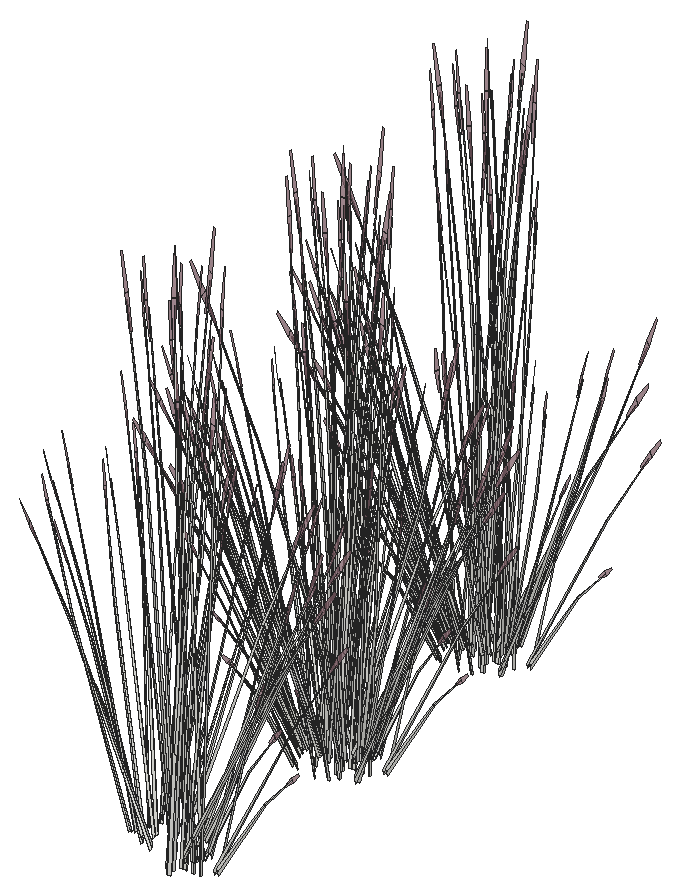
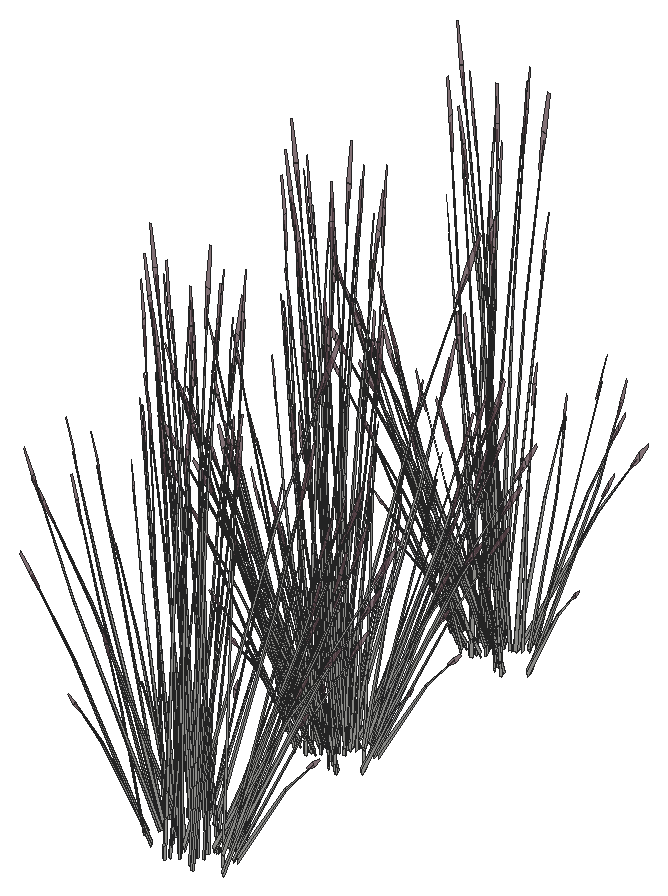
# SketchUp Ruby script. Lengths in inches.
U = 1.inch
M = Sketchup.active_model
def pt(a) = Geom::Point3d.new(a.map { |v| v * U })
def face(e, loops, mat)
  f = e.add_face(loops[0].map { |a| pt(a) })
  loops[1..].each { |l| e.add_face(l.map { |a| pt(a) }).erase! }
  f.material = f.back_material = mat if mat
  f
end
# faces: each face lists its corners as indices into pts; further lists are holes
def faces(e, pts, list, mat = nil) = list.each { |f| face(e, (f[0].is_a?(Array) ? f : [f]).map { |l| l.map { |i| pts[i] } }, mat) }
# xy, xz, yz: faces in a plane at the given z, y or x. An outline is a flat list of corners, or four numbers for a rectangle; further outlines are holes
def ring(l) = l.size == 4 ? [[l[0], l[1]], [l[2], l[1]], [l[2], l[3]], [l[0], l[3]]] : l.each_slice(2).to_a
def flat(e, list, mat, &to3) = list.each { |f| face(e, (f[0].is_a?(Array) ? f : [f]).map { |l| ring(l).map { |u, v| to3.(u, v) } }, mat) }
def xy(e, z, list, mat = nil) = flat(e, list, mat) { |x, y| [x, y, z] }
def xz(e, y, list, mat = nil) = flat(e, list, mat) { |x, z| [x, y, z] }
def yz(e, x, list, mat = nil) = flat(e, list, mat) { |y, z| [x, y, z] }
def lines(e, pts, list) = list.each { |a, b| e.add_line(pt(pts[a]), pt(pts[b])) }
# prism: a flat outline (further loops are holes) pulled along v
def prism(e, loops, v, mat = nil)
  f = face(e, loops, mat); d = Geom::Vector3d.new(v.map { |x| x * U })
  f.pushpull(f.normal.samedirection?(d) ? d.length : -d.length)
end
def box(e, o, s, mat = nil) = prism(e, [[o, [o[0] + s[0], o[1], o[2]], [o[0] + s[0], o[1] + s[1], o[2]], [o[0], o[1] + s[1], o[2]]]], [0, 0, s[2]], mat)
def at(x, y, z, deg = 0) = Geom::Transformation.translation(pt([x, y, z])) * Geom::Transformation.rotation(ORIGIN, Z_AXIS, deg.degrees)
def axes(o, x, y, z) = Geom::Transformation.new([*x, 0, *y, 0, *z, 0, *pt(o).to_a, 1])
def part(name) = M.definitions.add(name)
# library, detail: a bought-in or finely detailed component or shape, given as its bounding box
def library(name, o, s) = part(name).tap { |d| box(d.entities, o, s) }
def detail(e, o, s) = box(e.add_group.entities, o, s)
def put(e, d, t, mat = nil) = e.add_instance(d, t).tap { |i| i.material = mat if mat }
def group(e, t, mat = nil) = e.add_group.tap { |g| g.transformation = t; g.material = mat if mat }.entities
root = M.entities
M.materials.add("LightPink_Translucent").color = [144, 107, 117]
M.materials["LightPink_Translucent"].alpha = 0.75
c1 = part("blade")
p = [[2.15,0.21,22],[0,0.17,0],[0.09,0.45,0],[2.18,0.31,22],[2.29,0.31,22],[0.38,0.45,0],
  [2.48,0.24,33],[2.49,0.24,33],[2.48,0.22,33]]
faces(c1.entities,p,[[0,1,2,3],[4,5,2,3],[6,3,4,7],[8,0,3,6]])
c2 = part("seeds")
p = [[0.3,-0.1,1.38],[-0.01,-0.03,1.59],[-0.01,-0.03,0.03],[0.14,-0.07,-0.07],[0.29,-0.03,3],[0.15,0.01,3.11]]
faces(c2.entities,p,[[0,1,2,3],[1,0,4,5]],"LightPink_Translucent")
c3 = part("blade with seeds")
put(c3.entities,c1,at(0,0,0))
put(c3.entities,c2,axes([2.4,0.25,30.99],[1.5799,-0.05474,1.17369],[-0.12525,1.92788,0.29478],[-0.07173,-0.02425,1.56792]))
put(root,c3,axes([409,146.9,257.72],[-0.45644,-0.51287,0.44739],[0.69137,-0.36116,-0.21531],[0.14771,0.06346,1.43643]))
put(root,c3,axes([407.55,149.22,257.47],[0.81646,-0.16218,0.17642],[0.20161,0.60355,0.35086],[-0.07282,-0.08794,1.60407]))
put(root,c3,axes([412.28,148.01,259.53],[0.63144,0.17046,-0.35414],[-0.18417,0.49731,0.4572],[0.25423,-0.0456,0.87481]))
put(root,c3,axes([404.86,147.22,259.53],[-0.63144,-0.17046,-0.35414],[0.18417,-0.49731,0.4572],[-0.25423,0.0456,0.87481]))
put(root,c3,axes([410.06,146.12,257.47],[-0.81646,0.16218,0.17642],[-0.20161,-0.60355,0.35086],[0.07282,0.08794,1.60407]))
put(root,c3,axes([410.5625,147.39,258.875],[-0.31515,0.01384,1.71376],[0.20907,-0.5998,0.13857],[0.44912,0.0371,0.73262]))
put(root,c3,axes([409.54,147.28,257.38],[-0.96033,-0.12874,0.49198],[0.19544,-0.7271,0.19306],[0.14034,0.07021,1.70813]))
put(root,c3,axes([408.3,148.58,257.62],[-0.14658,0.54532,0.1448],[-0.71613,-0.09466,-0.41347],[-0.13033,-0.05599,1.26744]))
put(root,c3,axes([409.98,149.25,257.47],[0.21949,-0.60727,0.17642],[0.8032,0.17185,0.35086],[-0.13875,0.00296,1.60407]))
put(root,c3,axes([406.78,147.13,258.34],[0.21597,-0.08839,1.77064],[0.07448,0.61717,0.13857],[-0.4678,0.08189,0.63284]))
put(root,c3,axes([411.23,147.7,257.47],[-0.59697,-0.44509,0.17642],[0.60159,-0.4317,0.35086],[-0.06593,0.0909,1.60407]))
put(root,c3,axes([413.62,148.11,257.77],[-0.46945,0.10088,1.1486],[0.22097,-0.4169,0.84392],[0.24904,0.02853,0.25299]))
put(root,c3,axes([407.28,149.53,257.48],[0.7111,0.30552,0.49651],[-0.42504,0.54784,0],[-0.16196,-0.06958,1.57504]))
put(root,c3,axes([409.79,147.41,257.72],[0.36864,-0.55059,0.44739],[0.76598,0.26498,-0.21531],[0,0.12692,1.43643]))
put(root,c3,axes([405.29,147.47,259.68],[-0.20584,0.55581,-0.51099],[-0.70573,-0.19051,-0.3958],[-0.28414,0.05097,0.97773]))
put(root,c3,axes([412.81,149.39,258.93],[-0.14542,-0.51365,-0.03492],[0.68734,-0.11809,-0.15832],[0.14353,0.03256,0.52218]))
put(root,c3,axes([411.73,147.72,257.48],[0,-0.61104,0.49651],[0.85008,0,0],[0,0.13917,1.57504]))
put(root,c3,axes([409.6,148.18,257.72],[0.82508,-0.03772,0.44739],[0.07462,0.62614,-0.21531],[-0.14771,0.06346,1.43643]))
put(root,c3,axes([410.11,147.54,257.62],[0.70791,-0.1782,0.1448],[0.24791,0.50885,-0.41347],[0,0.11199,1.26744]))
put(root,c3,axes([412.74,148.78,257.59],[-0.18299,-0.15028,1.43002],[0.23809,-0.49714,-0.30754],[0.37023,0.06735,0.61141]))
put(root,c3,axes([409.61,148.45,257.62],[0.56134,0.36712,0.1448],[-0.46823,0.41419,-0.41347],[-0.13033,0.05599,1.26744]))
put(root,c3,axes([405.27,147.76,258.875],[0.26363,-0.12925,1.71376],[0.22195,0.59723,0.13857],[-0.41388,0.13498,0.73262]))
put(root,c3,axes([411.0625,149.08,259.98],[0.75952,0.01471,-0.71045],[-0.05101,0.61953,0.08574],[0.32177,0.06538,1.00501]))
put(root,c3,axes([410.21,149.58,257.48],[0.7111,-0.30552,0.49651],[0.42504,0.54784,0],[-0.16196,0.06958,1.57504]))
put(root,c3,axes([404.45,148.77,257.59],[0.26405,0.05016,1.43002],[0.17019,0.51235,-0.30754],[-0.35868,0.0959,0.61141]))
put(root,c3,axes([403.9,149.85,257.77],[0.31665,-0.27694,1.1486],[0.12495,0.43841,0.84392],[-0.22883,0.0785,0.25299]))
put(root,c3,axes([411.52,149.34,259.53],[0.43232,0.38257,-0.35414],[-0.49364,0.36215,0.4572],[0.25081,0.0551,0.87481]))
put(root,c3,axes([405.09,148.65,259.53],[-0.66138,0.08733,-0.35414],[-0.17464,-0.49921,0.4572],[-0.18953,0.13408,0.87481]))
put(root,c3,axes([409.97,148.35,258.875],[-0.28223,-0.10528,1.71376],[0.58406,-0.44165,0.13857],[0.36402,0.19924,0.73262]))
put(root,c3,axes([411.01,149.55,257.77],[-0.4278,-0.1757,1.1486],[0.5524,-0.17852,0.84392],[0.14899,0.15122,0.25299]))
put(root,c3,axes([406.23,148.16,258.875],[0.18977,-0.18775,1.71376],[0.47917,0.50677,0.13857],[-0.32866,0.23079,0.73262]))
put(root,c3,axes([405.64,148.71,259.68],[0.19519,0.55794,-0.51099],[-0.73919,0.0976,-0.3958],[-0.21183,0.14986,0.97773]))
put(root,c3,axes([409.97,147.58,257.84],[-0.02076,-0.57531,1.41272],[0.93937,0.14913,0.59816],[-0.22217,0.31481,1.3335]))
put(root,c3,axes([410.04,149.8,259.68],[0.74975,-0.14525,-0.51099],[0.13115,0.55007,-0.3958],[0.20138,0.15763,0.97773]))
put(root,c3,axes([411.08,150.35,257.67],[-0.48723,-0.01916,1.0506],[0.32177,-0.40701,0.58006],[0.19248,0.1446,0.8241]))
put(root,c3,axes([406.09,148.62,258.875],[0.14147,-0.21002,1.71376],[0.59349,0.43464,0.13857],[-0.26773,0.27089,0.73262]))
put(root,c3,axes([409.49,149.37,257.59],[0.01341,-0.20255,1.43002],[0.64074,-0.22625,-0.30754],[0.1978,0.24243,0.61141]))
put(root,c3,axes([406.25,149.81,259.53],[-0.5141,0.32171,-0.35414],[-0.48666,-0.36734,0.4572],[-0.07405,0.18664,0.87481]))
put(root,c3,axes([406.58,151.06,257.77],[-0.01966,-0.36332,1.1486],[0.49135,0.25914,0.84392],[-0.09663,0.17317,0.25299]))
put(root,c3,axes([406.77,149.65,260],[0.54391,0.41056,-0.5672],[-0.57458,0.35956,-0.43934],[-0.08276,0.2086,1.08528]))
put(root,c3,axes([406.18,150.27,257.82],[0.69024,-0.1082,0.06507],[0.15868,0.43593,-0.86304],[-0.04376,0.22067,0.7736]))
put(root,c3,axes([408.38,150.05,259.68],[0.7469,0.15318,-0.51099],[-0.25601,0.52518,-0.3958],[0.06849,0.21144,0.97773]))
put(root,c3,axes([408.8,148.97,258.875],[-0.17368,-0.19618,1.71376],[0.80256,-0.16516,0.13857],[0.18139,0.30799,0.73262]))
put(root,c3,axes([408.04,150.375,259.53],[-0.22906,0.4699,-0.35414],[-0.66828,-0.13705,0.4572],[0.06128,0.18919,0.87481]))
put(root,c3,axes([406.6,149.47,260.34],[-0.01977,0.56521,-0.7886],[-0.83252,-0.03796,0.09517],[-0.08786,0.23945,1.11556]))
put(root,c3,axes([407.38,149.06,258.875],[-0.0186,-0.23452,1.71376],[0.80601,0.15558,0.13857],[-0.04985,0.33422,0.73262]))
put(root,c3,axes([408.11,149.95,259.98],[0.36264,0.49684,-0.71045],[-0.74649,0.27689,0.08574],[0.0848,0.24006,1.00501]))
put(root,c3,axes([406.01,150.73,257.59],[0.23977,-0.09639,1.43002],[0.59198,0.29065,-0.30754],[-0.1762,0.25149,0.61141]))
put(root,c3,axes([406.32,150.26,258.36],[0.01669,-0.31544,1.54345],[0.75083,0.16661,0.21329],[-0.06506,0.33618,0.72882]))
put(root,c3,axes([407.26,167.72,258.875],[0.17368,0.19618,1.71376],[-0.80256,0.16516,0.13857],[-0.18139,-0.30799,0.73262]))
put(root,c3,axes([410.38,167.44,257.59],[-0.21597,0.12368,1.43002],[-0.64681,-0.21647,-0.30754],[0.1199,-0.26922,0.61141]))
put(root,c3,axes([409.4,167.87,259.98],[-0.36264,-0.49684,-0.71045],[0.74649,-0.27689,0.08574],[-0.0848,-0.24006,1.00501]))
put(root,c3,axes([407.04,167.2,257.59],[-0.04601,0.19989,1.43002],[-0.67263,0.16733,-0.30754],[-0.15723,-0.25836,0.61141]))
put(root,c3,axes([410.91,168.35,259.98],[0.01977,-0.56521,-0.71045],[0.83252,0.03796,0.08574],[0.08786,-0.23945,1.00501]))
put(root,c3,axes([409.46,167.44,259.53],[0.22906,-0.4699,-0.35414],[0.66828,0.13705,0.4572],[-0.06128,-0.18919,0.87481]))
put(root,c3,axes([409.97,168.07,258.875],[-0.14147,0.21002,1.71376],[-0.59349,-0.43464,0.13857],[0.26773,-0.27089,0.73262]))
put(root,c3,axes([409.125,167.77,259.68],[-0.7469,-0.15318,-0.51099],[0.25601,-0.52518,-0.3958],[-0.06849,-0.21144,0.97773]))
put(root,c3,axes([409.59,166.45,257.77],[0.09747,0.35631,1.1486],[-0.54071,-0.19735,0.84392],[0.05818,-0.18244,0.25299]))
put(root,c3,axes([410.74,168.16,259.68],[-0.54391,-0.41056,-0.51099],[0.57458,-0.35956,-0.3958],[0.08276,-0.2086,0.97773]))
put(root,c3,axes([411.25,168.01,259.53],[0.5141,-0.32171,-0.35414],[0.48666,0.36734,0.4572],[0.07405,-0.18664,0.87481]))
put(root,c3,axes([406.81,166.88,257.77],[0.39634,0.21267,1.1486],[-0.57721,0.12784,0.84392],[-0.1235,-0.16344,0.25299]))
put(root,c3,axes([407.76,168.01,259.98],[-0.64788,-0.29534,-0.71045],[0.46044,-0.51755,0.08574],[-0.23473,-0.17635,1.00501]))
put(root,c3,axes([407.54,167.62,259.53],[-0.11735,-0.49217,-0.35414],[0.67083,-0.12996,0.4572],[-0.18018,-0.14104,0.87481]))
put(root,c3,axes([406.09,168.33,258.875],[0.28223,0.10528,1.71376],[-0.58406,0.44165,0.13857],[-0.36402,-0.19924,0.73262]))
put(root,c3,axes([407.46,168.02,259.68],[-0.74975,0.14525,-0.51099],[-0.13115,-0.55007,-0.3958],[-0.20138,-0.15763,0.97773]))
put(root,c3,axes([411.89,169.33,259.98],[0.39688,-0.48213,-0.71045],[0.69548,0.34264,0.08574],[0.23697,-0.17468,1.00501]))
put(root,c3,axes([411.87,169.11,259.68],[-0.19519,-0.55794,-0.51099],[0.73919,-0.0976,-0.3958],[0.21183,-0.14986,0.97773]))
put(root,c3,axes([409.3125,171.35,258.33],[0.65659,0.2464,1.51261],[-0.64324,0.53082,0.59816],[-0.28812,-0.31461,1.26806]))
put(root,c3,axes([412.46,168.89,257.59],[-0.27143,-0.0181,1.43002],[-0.27808,-0.48551,-0.30754],[0.33346,-0.13735,0.61141]))
put(root,c3,axes([412.77,168,257.77],[-0.25308,0.31105,1.1486],[-0.21753,-0.4179,0.84392],[0.20902,-0.10472,0.25299]))
put(root,c3,axes([412.41,169.17,259.53],[0.66138,-0.08733,-0.35414],[0.17464,0.49921,0.4572],[0.18953,-0.13408,0.87481]))
put(root,c3,axes([405.98,168.48,259.53],[-0.43232,-0.38257,-0.35414],[0.49364,-0.36215,0.4572],[-0.25081,-0.0551,0.87481]))
put(root,c3,axes([405.83,168.89,257.59],[0.14835,0.17012,1.43002],[-0.34183,0.46242,-0.30754],[-0.351,-0.11053,0.61141]))
put(root,c3,axes([406.44,168.74,259.98],[-0.75952,-0.01471,-0.71045],[0.05101,-0.61953,0.08574],[-0.32177,-0.06538,1.00501]))
put(root,c3,axes([408.65,170.17,257.43],[0.8561,0.29616,0.24065],[-0.41201,0.61537,0.50002],[0,-0.14185,1.60543]))
put(root,c3,axes([406.1875,168.86,259.68],[-0.55171,0.40476,-0.51099],[-0.48318,-0.42758,-0.3958],[-0.28031,-0.06159,0.97773]))
put(root,c3,axes([404.95,169.4,257.77],[0.48508,-0.04372,1.1486],[-0.3077,0.38525,0.84392],[-0.23971,-0.05779,0.25299]))
put(root,c3,axes([408.375,169.75,257.72],[-0.82508,0.03772,0.44739],[-0.07462,-0.62614,-0.21531],[0.14771,-0.06346,1.43643]))
put(root,c3,axes([406.24,170.21,257.48],[0,0.61104,0.49651],[-0.85008,0,0],[0,-0.13917,1.57504]))
put(root,c3,axes([412.21,170.35,259.68],[0.20584,-0.55581,-0.51099],[0.70573,0.19051,-0.3958],[0.28414,-0.05097,0.97773]))
put(root,c3,axes([405.5,169.29,258.875],[0.31515,-0.01384,1.71376],[-0.20907,0.5998,0.13857],[-0.44912,-0.0371,0.73262]))
put(root,c3,axes([408.18,170.52,257.72],[-0.36864,0.55059,0.44739],[-0.76598,-0.26498,-0.21531],[0,-0.12692,1.43643]))
put(root,c3,axes([410.69,168.4,257.48],[-0.7111,-0.30552,0.49651],[0.42504,-0.54784,0],[0.16196,0.06958,1.57504]))
put(root,c3,axes([412.08,170.55,259.98],[0.66765,-0.26986,-0.71045],[0.37208,0.55551,0.08574],[0.32259,-0.0631,1.00501]))
put(root,c3,axes([407.99,168.68,257.47],[-0.21949,0.60727,0.17642],[-0.8032,-0.17185,0.35086],[0.13875,-0.00296,1.60407]))
put(root,c3,axes([409.67,169.35,257.62],[0.14658,-0.54532,0.1448],[0.71613,0.09466,-0.41347],[0.13033,0.05599,1.26744]))
put(root,c3,axes([409.36,169.5,257.72],[-0.45644,-0.51287,0.44739],[0.69137,-0.36116,-0.21531],[0.14771,0.06346,1.43643]))
put(root,c3,axes([407.91,171.8125,257.47],[0.81646,-0.16218,0.17642],[0.20161,0.60355,0.35086],[-0.07282,-0.08794,1.60407]))
put(root,c3,axes([412.64,170.6,259.53],[0.63144,0.17046,-0.35414],[-0.18417,0.49731,0.4572],[0.25423,-0.0456,0.87481]))
put(root,c3,axes([405.22,169.81,259.53],[-0.63144,-0.17046,-0.35414],[0.18417,-0.49731,0.4572],[-0.25423,0.0456,0.87481]))
put(root,c3,axes([410.42,168.71,257.47],[-0.81646,0.16218,0.17642],[-0.20161,-0.60355,0.35086],[0.07282,0.08794,1.60407]))
put(root,c3,axes([410.92,169.99,258.875],[-0.31515,0.01384,1.71376],[0.20907,-0.5998,0.13857],[0.44912,0.0371,0.73262]))
put(root,c3,axes([409.9,169.875,257.38],[-0.96033,-0.12874,0.49198],[0.19544,-0.7271,0.19306],[0.14034,0.07021,1.70813]))
put(root,c3,axes([408.66,171.17,257.62],[-0.14658,0.54532,0.1448],[-0.71613,-0.09466,-0.41347],[-0.13033,-0.05599,1.26744]))
put(root,c3,axes([410.34,171.84,257.47],[0.21949,-0.60727,0.17642],[0.8032,0.17185,0.35086],[-0.13875,0.00296,1.60407]))
put(root,c3,axes([407.14,169.73,258.34],[0.21597,-0.08839,1.77064],[0.07448,0.61717,0.13857],[-0.4678,0.08189,0.63284]))
put(root,c3,axes([411.6,170.3,257.47],[-0.59697,-0.44509,0.17642],[0.60159,-0.4317,0.35086],[-0.06593,0.0909,1.60407]))
put(root,c3,axes([413.98,170.7,257.77],[-0.46945,0.10088,1.1486],[0.22097,-0.4169,0.84392],[0.24904,0.02853,0.25299]))
put(root,c3,axes([407.65,172.12,257.48],[0.7111,0.30552,0.49651],[-0.42504,0.54784,0],[-0.16196,-0.06958,1.57504]))
put(root,c3,axes([410.15,170.01,257.72],[0.36864,-0.55059,0.44739],[0.76598,0.26498,-0.21531],[0,0.12692,1.43643]))
put(root,c3,axes([405.65,170.0625,259.68],[-0.20584,0.55581,-0.51099],[-0.70573,-0.19051,-0.3958],[-0.28414,0.05097,0.97773]))
put(root,c3,axes([413.17,171.99,258.93],[-0.14542,-0.51365,-0.03492],[0.68734,-0.11809,-0.15832],[0.14353,0.03256,0.52218]))
put(root,c3,axes([412.09,170.3125,257.48],[0,-0.61104,0.49651],[0.85008,0,0],[0,0.13917,1.57504]))
put(root,c3,axes([409.96,170.77,257.72],[0.82508,-0.03772,0.44739],[0.07462,0.62614,-0.21531],[-0.14771,0.06346,1.43643]))
put(root,c3,axes([410.47,170.13,257.62],[0.70791,-0.1782,0.1448],[0.24791,0.50885,-0.41347],[0,0.11199,1.26744]))
put(root,c3,axes([413.1,171.37,257.59],[-0.18299,-0.15028,1.43002],[0.23809,-0.49714,-0.30754],[0.37023,0.06735,0.61141]))
put(root,c3,axes([409.97,171.04,257.62],[0.56134,0.36712,0.1448],[-0.46823,0.41419,-0.41347],[-0.13033,0.05599,1.26744]))
put(root,c3,axes([405.63,170.35,258.875],[0.26363,-0.12925,1.71376],[0.22195,0.59723,0.13857],[-0.41388,0.13498,0.73262]))
put(root,c3,axes([411.42,171.67,259.98],[0.75952,0.01471,-0.71045],[-0.05101,0.61953,0.08574],[0.32177,0.06538,1.00501]))
put(root,c3,axes([410.57,172.17,257.48],[0.7111,-0.30552,0.49651],[0.42504,0.54784,0],[-0.16196,0.06958,1.57504]))
put(root,c3,axes([404.81,171.37,257.59],[0.26405,0.05016,1.43002],[0.17019,0.51235,-0.30754],[-0.35868,0.0959,0.61141]))
put(root,c3,axes([404.26,172.44,257.77],[0.31665,-0.27694,1.1486],[0.12495,0.43841,0.84392],[-0.22883,0.0785,0.25299]))
put(root,c3,axes([411.88,171.93,259.53],[0.43232,0.38257,-0.35414],[-0.49364,0.36215,0.4572],[0.25081,0.0551,0.87481]))
put(root,c3,axes([405.45,171.24,259.53],[-0.66138,0.08733,-0.35414],[-0.17464,-0.49921,0.4572],[-0.18953,0.13408,0.87481]))
put(root,c3,axes([410.33,170.95,258.875],[-0.28223,-0.10528,1.71376],[0.58406,-0.44165,0.13857],[0.36402,0.19924,0.73262]))
put(root,c3,axes([411.37,172.15,257.77],[-0.4278,-0.1757,1.1486],[0.5524,-0.17852,0.84392],[0.14899,0.15122,0.25299]))
put(root,c3,axes([406.59,170.75,258.875],[0.18977,-0.18775,1.71376],[0.47917,0.50677,0.13857],[-0.32866,0.23079,0.73262]))
put(root,c3,axes([406,171.3,259.68],[0.19519,0.55794,-0.51099],[-0.73919,0.0976,-0.3958],[-0.21183,0.14986,0.97773]))
put(root,c3,axes([410.33,170.17,257.84],[-0.02076,-0.57531,1.41272],[0.93937,0.14913,0.59816],[-0.22217,0.31481,1.3335]))
put(root,c3,axes([410.41,172.39,259.68],[0.74975,-0.14525,-0.51099],[0.13115,0.55007,-0.3958],[0.20138,0.15763,0.97773]))
put(root,c3,axes([411.44,172.95,257.67],[-0.48723,-0.01916,1.0506],[0.32177,-0.40701,0.58006],[0.19248,0.1446,0.8241]))
put(root,c3,axes([406.45,171.21,258.875],[0.14147,-0.21002,1.71376],[0.59349,0.43464,0.13857],[-0.26773,0.27089,0.73262]))
put(root,c3,axes([409.85,171.96,257.59],[0.01341,-0.20255,1.43002],[0.64074,-0.22625,-0.30754],[0.1978,0.24243,0.61141]))
put(root,c3,axes([406.62,172.4,259.53],[-0.5141,0.32171,-0.35414],[-0.48666,-0.36734,0.4572],[-0.07405,0.18664,0.87481]))
put(root,c3,axes([406.94,173.65,257.77],[-0.01966,-0.36332,1.1486],[0.49135,0.25914,0.84392],[-0.09663,0.17317,0.25299]))
put(root,c3,axes([407.13,172.25,260],[0.54391,0.41056,-0.5672],[-0.57458,0.35956,-0.43934],[-0.08276,0.2086,1.08528]))
put(root,c3,axes([406.54,172.86,257.82],[0.69024,-0.1082,0.06507],[0.15868,0.43593,-0.86304],[-0.04376,0.22067,0.7736]))
put(root,c3,axes([408.74,172.64,259.68],[0.7469,0.15318,-0.51099],[-0.25601,0.52518,-0.3958],[0.06849,0.21144,0.97773]))
put(root,c3,axes([409.16,171.5625,258.875],[-0.17368,-0.19618,1.71376],[0.80256,-0.16516,0.13857],[0.18139,0.30799,0.73262]))
put(root,c3,axes([408.4,172.97,259.53],[-0.22906,0.4699,-0.35414],[-0.66828,-0.13705,0.4572],[0.06128,0.18919,0.87481]))
put(root,c3,axes([406.96,172.06,260.34],[-0.01977,0.56521,-0.7886],[-0.83252,-0.03796,0.09517],[-0.08786,0.23945,1.11556]))
put(root,c3,axes([407.75,171.66,258.875],[-0.0186,-0.23452,1.71376],[0.80601,0.15558,0.13857],[-0.04985,0.33422,0.73262]))
put(root,c3,axes([408.47,172.55,259.98],[0.36264,0.49684,-0.71045],[-0.74649,0.27689,0.08574],[0.0848,0.24006,1.00501]))
put(root,c3,axes([406.37,173.33,257.59],[0.23977,-0.09639,1.43002],[0.59198,0.29065,-0.30754],[-0.1762,0.25149,0.61141]))
put(root,c3,axes([406.68,172.86,258.36],[0.01669,-0.31544,1.54345],[0.75083,0.16661,0.21329],[-0.06506,0.33618,0.72882]))
put(root,c3,axes([405.24,189.85,258.875],[0.17368,0.19618,1.71376],[-0.80256,0.16516,0.13857],[-0.18139,-0.30799,0.73262]))
put(root,c3,axes([408.36,189.57,257.59],[-0.21597,0.12368,1.43002],[-0.64681,-0.21647,-0.30754],[0.1199,-0.26922,0.61141]))
put(root,c3,axes([407.38,190,259.98],[-0.36264,-0.49684,-0.71045],[0.74649,-0.27689,0.08574],[-0.0848,-0.24006,1.00501]))
put(root,c3,axes([405.02,189.33,257.59],[-0.04601,0.19989,1.43002],[-0.67263,0.16733,-0.30754],[-0.15723,-0.25836,0.61141]))
put(root,c3,axes([408.89,190.48,259.98],[0.01977,-0.56521,-0.71045],[0.83252,0.03796,0.08574],[0.08786,-0.23945,1.00501]))
put(root,c3,axes([407.45,189.57,259.53],[0.22906,-0.4699,-0.35414],[0.66828,0.13705,0.4572],[-0.06128,-0.18919,0.87481]))
put(root,c3,axes([407.95,190.2,258.875],[-0.14147,0.21002,1.71376],[-0.59349,-0.43464,0.13857],[0.26773,-0.27089,0.73262]))
put(root,c3,axes([407.11,189.9,259.68],[-0.7469,-0.15318,-0.51099],[0.25601,-0.52518,-0.3958],[-0.06849,-0.21144,0.97773]))
put(root,c3,axes([407.57,188.58,257.77],[0.09747,0.35631,1.1486],[-0.54071,-0.19735,0.84392],[0.05818,-0.18244,0.25299]))
put(root,c3,axes([408.72,190.29,259.68],[-0.54391,-0.41056,-0.51099],[0.57458,-0.35956,-0.3958],[0.08276,-0.2086,0.97773]))
put(root,c3,axes([409.23,190.14,259.53],[0.5141,-0.32171,-0.35414],[0.48666,0.36734,0.4572],[0.07405,-0.18664,0.87481]))
put(root,c3,axes([404.79,189.01,257.77],[0.39634,0.21267,1.1486],[-0.57721,0.12784,0.84392],[-0.1235,-0.16344,0.25299]))
put(root,c3,axes([405.74,190.14,259.98],[-0.64788,-0.29534,-0.71045],[0.46044,-0.51755,0.08574],[-0.23473,-0.17635,1.00501]))
put(root,c3,axes([405.52,189.75,259.53],[-0.11735,-0.49217,-0.35414],[0.67083,-0.12996,0.4572],[-0.18018,-0.14104,0.87481]))
put(root,c3,axes([404.08,190.46,258.875],[0.28223,0.10528,1.71376],[-0.58406,0.44165,0.13857],[-0.36402,-0.19924,0.73262]))
put(root,c3,axes([405.44,190.15,259.68],[-0.74975,0.14525,-0.51099],[-0.13115,-0.55007,-0.3958],[-0.20138,-0.15763,0.97773]))
put(root,c3,axes([409.87,191.47,259.98],[0.39688,-0.48213,-0.71045],[0.69548,0.34264,0.08574],[0.23697,-0.17468,1.00501]))
put(root,c3,axes([409.85,191.24,259.68],[-0.19519,-0.55794,-0.51099],[0.73919,-0.0976,-0.3958],[0.21183,-0.14986,0.97773]))
put(root,c3,axes([407.29,193.48,258.33],[0.65659,0.2464,1.51261],[-0.64324,0.53082,0.59816],[-0.28812,-0.31461,1.26806]))
put(root,c3,axes([410.44,191.02,257.59],[-0.27143,-0.0181,1.43002],[-0.27808,-0.48551,-0.30754],[0.33346,-0.13735,0.61141]))
put(root,c3,axes([410.76,190.13,257.77],[-0.25308,0.31105,1.1486],[-0.21753,-0.4179,0.84392],[0.20902,-0.10472,0.25299]))
put(root,c3,axes([410.39,191.3,259.53],[0.66138,-0.08733,-0.35414],[0.17464,0.49921,0.4572],[0.18953,-0.13408,0.87481]))
put(root,c3,axes([403.97,190.61,259.53],[-0.43232,-0.38257,-0.35414],[0.49364,-0.36215,0.4572],[-0.25081,-0.0551,0.87481]))
put(root,c3,axes([403.81,191.02,257.59],[0.14835,0.17012,1.43002],[-0.34183,0.46242,-0.30754],[-0.351,-0.11053,0.61141]))
put(root,c3,axes([404.42,190.87,259.98],[-0.75952,-0.01471,-0.71045],[0.05101,-0.61953,0.08574],[-0.32177,-0.06538,1.00501]))
put(root,c3,axes([406.63,192.3,257.43],[0.8561,0.29616,0.24065],[-0.41201,0.61537,0.50002],[0,-0.14185,1.60543]))
put(root,c3,axes([404.17,190.99,259.68],[-0.55171,0.40476,-0.51099],[-0.48318,-0.42758,-0.3958],[-0.28031,-0.06159,0.97773]))
put(root,c3,axes([402.93,191.53,257.77],[0.48508,-0.04372,1.1486],[-0.3077,0.38525,0.84392],[-0.23971,-0.05779,0.25299]))
put(root,c3,axes([406.36,191.89,257.72],[-0.82508,0.03772,0.44739],[-0.07462,-0.62614,-0.21531],[0.14771,-0.06346,1.43643]))
put(root,c3,axes([404.23,192.34,257.48],[0,0.61104,0.49651],[-0.85008,0,0],[0,-0.13917,1.57504]))
put(root,c3,axes([410.19,192.48,259.68],[0.20584,-0.55581,-0.51099],[0.70573,0.19051,-0.3958],[0.28414,-0.05097,0.97773]))
put(root,c3,axes([403.48,191.43,258.875],[0.31515,-0.01384,1.71376],[-0.20907,0.5998,0.13857],[-0.44912,-0.0371,0.73262]))
put(root,c3,axes([406.16,192.65,257.72],[-0.36864,0.55059,0.44739],[-0.76598,-0.26498,-0.21531],[0,-0.12692,1.43643]))
put(root,c3,axes([408.67,190.54,257.48],[-0.7111,-0.30552,0.49651],[0.42504,-0.54784,0],[0.16196,0.06958,1.57504]))
put(root,c3,axes([410.06,192.68,259.98],[0.66765,-0.26986,-0.71045],[0.37208,0.55551,0.08574],[0.32259,-0.0631,1.00501]))
put(root,c3,axes([405.97,190.8125,257.47],[-0.21949,0.60727,0.17642],[-0.8032,-0.17185,0.35086],[0.13875,-0.00296,1.60407]))
put(root,c3,axes([407.65,191.49,257.62],[0.14658,-0.54532,0.1448],[0.71613,0.09466,-0.41347],[0.13033,0.05599,1.26744]))
put(root,c3,axes([407.34,191.63,257.72],[-0.45644,-0.51287,0.44739],[0.69137,-0.36116,-0.21531],[0.14771,0.06346,1.43643]))
put(root,c3,axes([405.89,193.94,257.47],[0.81646,-0.16218,0.17642],[0.20161,0.60355,0.35086],[-0.07282,-0.08794,1.60407]))
put(root,c3,axes([410.625,192.73,259.53],[0.63144,0.17046,-0.35414],[-0.18417,0.49731,0.4572],[0.25423,-0.0456,0.87481]))
put(root,c3,axes([403.2,191.94,259.53],[-0.63144,-0.17046,-0.35414],[0.18417,-0.49731,0.4572],[-0.25423,0.0456,0.87481]))
put(root,c3,axes([408.4,190.84,257.47],[-0.81646,0.16218,0.17642],[-0.20161,-0.60355,0.35086],[0.07282,0.08794,1.60407]))
put(root,c3,axes([408.9,192.12,258.875],[-0.31515,0.01384,1.71376],[0.20907,-0.5998,0.13857],[0.44912,0.0371,0.73262]))
put(root,c3,axes([407.88,192.01,257.38],[-0.96033,-0.12874,0.49198],[0.19544,-0.7271,0.19306],[0.14034,0.07021,1.70813]))
put(root,c3,axes([406.65,193.3,257.62],[-0.14658,0.54532,0.1448],[-0.71613,-0.09466,-0.41347],[-0.13033,-0.05599,1.26744]))
put(root,c3,axes([408.32,193.98,257.47],[0.21949,-0.60727,0.17642],[0.8032,0.17185,0.35086],[-0.13875,0.00296,1.60407]))
put(root,c3,axes([405.125,191.86,258.34],[0.21597,-0.08839,1.77064],[0.07448,0.61717,0.13857],[-0.4678,0.08189,0.63284]))
put(root,c3,axes([409.58,192.43,257.47],[-0.59697,-0.44509,0.17642],[0.60159,-0.4317,0.35086],[-0.06593,0.0909,1.60407]))
put(root,c3,axes([411.96,192.83,257.77],[-0.46945,0.10088,1.1486],[0.22097,-0.4169,0.84392],[0.24904,0.02853,0.25299]))
put(root,c3,axes([405.63,194.25,257.48],[0.7111,0.30552,0.49651],[-0.42504,0.54784,0],[-0.16196,-0.06958,1.57504]))
put(root,c3,axes([408.13,192.14,257.72],[0.36864,-0.55059,0.44739],[0.76598,0.26498,-0.21531],[0,0.12692,1.43643]))
put(root,c3,axes([403.64,192.19,259.68],[-0.20584,0.55581,-0.51099],[-0.70573,-0.19051,-0.3958],[-0.28414,0.05097,0.97773]))
put(root,c3,axes([411.15,194.12,258.93],[-0.14542,-0.51365,-0.03492],[0.68734,-0.11809,-0.15832],[0.14353,0.03256,0.52218]))
put(root,c3,axes([410.07,192.44,257.48],[0,-0.61104,0.49651],[0.85008,0,0],[0,0.13917,1.57504]))
put(root,c3,axes([407.9375,192.9,257.72],[0.82508,-0.03772,0.44739],[0.07462,0.62614,-0.21531],[-0.14771,0.06346,1.43643]))
put(root,c3,axes([408.45,192.26,257.62],[0.70791,-0.1782,0.1448],[0.24791,0.50885,-0.41347],[0,0.11199,1.26744]))
put(root,c3,axes([411.08,193.5,257.59],[-0.18299,-0.15028,1.43002],[0.23809,-0.49714,-0.30754],[0.37023,0.06735,0.61141]))
put(root,c3,axes([407.95,193.17,257.62],[0.56134,0.36712,0.1448],[-0.46823,0.41419,-0.41347],[-0.13033,0.05599,1.26744]))
put(root,c3,axes([403.61,192.48,258.875],[0.26363,-0.12925,1.71376],[0.22195,0.59723,0.13857],[-0.41388,0.13498,0.73262]))
put(root,c3,axes([409.4,193.8,259.98],[0.75952,0.01471,-0.71045],[-0.05101,0.61953,0.08574],[0.32177,0.06538,1.00501]))
put(root,c3,axes([408.55,194.3,257.48],[0.7111,-0.30552,0.49651],[0.42504,0.54784,0],[-0.16196,0.06958,1.57504]))
put(root,c3,axes([402.79,193.5,257.59],[0.26405,0.05016,1.43002],[0.17019,0.51235,-0.30754],[-0.35868,0.0959,0.61141]))
